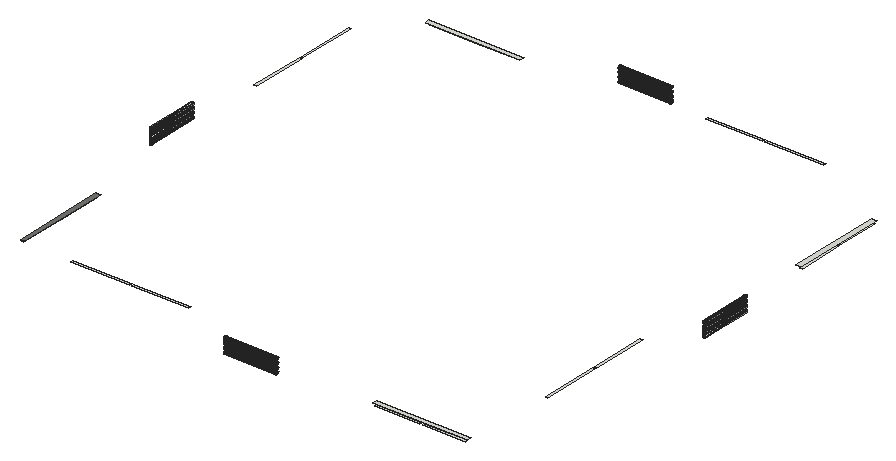
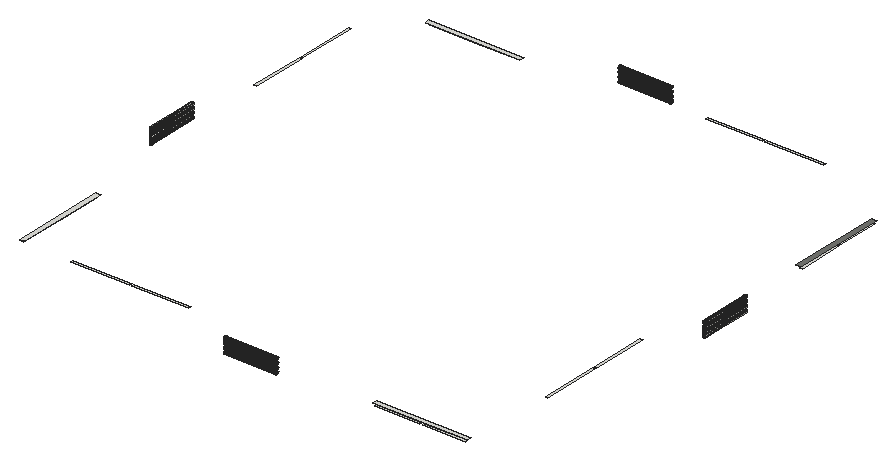
# SketchUp Ruby script. Lengths in inches.
U = 1.inch
M = Sketchup.active_model
def pt(a) = Geom::Point3d.new(a.map { |v| v * U })
def face(e, loops, mat)
  f = e.add_face(loops[0].map { |a| pt(a) })
  loops[1..].each { |l| e.add_face(l.map { |a| pt(a) }).erase! }
  f.material = f.back_material = mat if mat
  f
end
# faces: each face lists its corners as indices into pts; further lists are holes
def faces(e, pts, list, mat = nil) = list.each { |f| face(e, (f[0].is_a?(Array) ? f : [f]).map { |l| l.map { |i| pts[i] } }, mat) }
# xy, xz, yz: faces in a plane at the given z, y or x. An outline is a flat list of corners, or four numbers for a rectangle; further outlines are holes
def ring(l) = l.size == 4 ? [[l[0], l[1]], [l[2], l[1]], [l[2], l[3]], [l[0], l[3]]] : l.each_slice(2).to_a
def flat(e, list, mat, &to3) = list.each { |f| face(e, (f[0].is_a?(Array) ? f : [f]).map { |l| ring(l).map { |u, v| to3.(u, v) } }, mat) }
def xy(e, z, list, mat = nil) = flat(e, list, mat) { |x, y| [x, y, z] }
def xz(e, y, list, mat = nil) = flat(e, list, mat) { |x, z| [x, y, z] }
def yz(e, x, list, mat = nil) = flat(e, list, mat) { |y, z| [x, y, z] }
def lines(e, pts, list) = list.each { |a, b| e.add_line(pt(pts[a]), pt(pts[b])) }
# prism: a flat outline (further loops are holes) pulled along v
def prism(e, loops, v, mat = nil)
  f = face(e, loops, mat); d = Geom::Vector3d.new(v.map { |x| x * U })
  f.pushpull(f.normal.samedirection?(d) ? d.length : -d.length)
end
def box(e, o, s, mat = nil) = prism(e, [[o, [o[0] + s[0], o[1], o[2]], [o[0] + s[0], o[1] + s[1], o[2]], [o[0], o[1] + s[1], o[2]]]], [0, 0, s[2]], mat)
def at(x, y, z, deg = 0) = Geom::Transformation.translation(pt([x, y, z])) * Geom::Transformation.rotation(ORIGIN, Z_AXIS, deg.degrees)
def axes(o, x, y, z) = Geom::Transformation.new([*x, 0, *y, 0, *z, 0, *pt(o).to_a, 1])
def part(name) = M.definitions.add(name)
# library, detail: a bought-in or finely detailed component or shape, given as its bounding box
def library(name, o, s) = part(name).tap { |d| box(d.entities, o, s) }
def detail(e, o, s) = box(e.add_group.entities, o, s)
def put(e, d, t, mat = nil) = e.add_instance(d, t).tap { |i| i.material = mat if mat }
def group(e, t, mat = nil) = e.add_group.tap { |g| g.transformation = t; g.material = mat if mat }.entities
root = M.entities
M.materials.add("[Metal Seamed]").color = [118, 119, 115]
xy(root,1367.61,[[1161.2,84.8125,1285.04,90.8125],[1291.04,84.8125,1408.89,90.8125],[120,175.92,126,293.77],[120,299.77,126,423.61],[1494,1126.01,1500,1249.86],
  [1494,1255.86,1500,1373.7],[211.11,1458.8125,328.96,1464.8125],[334.96,1458.8125,458.8,1464.8125]])
xy(root,1373.61,[[1155.2,84.8125,1414.89,96.8125],[1488,1120.01,1500,1379.7],[205.11,1452.8125,464.8,1464.8125]])
xy(root,1373.61,[[120,169.92,132,429.61]],"[Metal Seamed]")
xy(root,1416.625,[[312.65,102.8125,473.9375,108.8125],[479.9375,102.8125,635.22,108.8125],[1476,277.47,1482,438.75],[1476,444.75,1482,600.03],[138,949.59,144,1104.875],
  [138,1110.875,144,1272.16],[984.78,1440.8125,1140.0625,1446.8125],[1146.0625,1440.8125,1307.35,1446.8125]])
p = [[922.01,48.34,1377.02],[922.01,47.38,1377.14],[778.64,47.38,1377.14],[778.64,48.34,1377.02],[922.01,49.29,1377.14],[778.64,49.29,1377.14],
  [83.53,662.8,1377.02],[82.57,662.8,1377.14],[82.57,806.17,1377.14],[83.53,806.17,1377.02],[84.48,662.8,1377.14],[84.48,806.17,1377.14],
  [1535.52,886.83,1377.14],[1536.47,886.83,1377.02],[1536.47,743.45,1377.02],[1535.52,743.45,1377.14],[1537.43,886.83,1377.14],[1537.43,743.45,1377.14],
  [697.99,1500.33,1377.14],[697.99,1501.28,1377.02],[841.36,1501.28,1377.02],[841.36,1500.33,1377.14],[697.99,1502.24,1377.14],[841.36,1502.24,1377.14],
  [922.01,46.5,1377.51],[778.64,46.5,1377.51],[922.01,50.18,1377.51],[778.64,50.18,1377.51],[81.68,662.8,1377.51],[81.68,806.17,1377.51],
  [85.37,662.8,1377.51],[85.37,806.17,1377.51],[1534.63,886.83,1377.51],[1534.63,743.45,1377.51],[1538.32,886.83,1377.51],[1538.32,743.45,1377.51],
  [697.99,1499.44,1377.51],[841.36,1499.44,1377.51],[697.99,1503.13,1377.51],[841.36,1503.13,1377.51],[922.01,45.73,1378.1],[778.64,45.73,1378.1],
  [922.01,50.95,1378.1],[778.64,50.95,1378.1],[80.92,662.8,1378.1],[80.92,806.17,1378.1],[86.13,662.8,1378.1],[86.13,806.17,1378.1],
  [1533.87,886.83,1378.1],[1533.87,743.45,1378.1],[1539.08,886.83,1378.1],[1539.08,743.45,1378.1],[697.99,1498.68,1378.1],[841.36,1498.68,1378.1],
  [697.99,1503.89,1378.1],[841.36,1503.89,1378.1],[922.01,45.15,1378.86],[778.64,45.15,1378.86],[922.01,51.53,1378.86],[778.64,51.53,1378.86],
  [80.33,662.8,1378.86],[80.33,806.17,1378.86],[86.72,662.8,1378.86],[86.72,806.17,1378.86],[1533.28,886.83,1378.86],[1533.28,743.45,1378.86],
  [1539.67,886.83,1378.86],[1539.67,743.45,1378.86],[697.99,1498.09,1378.86],[841.36,1498.09,1378.86],[697.99,1504.48,1378.86],[841.36,1504.48,1378.86],
  [922.01,44.78,1379.75],[778.64,44.78,1379.75],[922.01,51.9,1379.75],[778.64,51.9,1379.75],[79.97,662.8,1379.75],[79.97,806.17,1379.75],
  [87.09,662.8,1379.75],[87.09,806.17,1379.75],[1532.91,886.83,1379.75],[1532.91,743.45,1379.75],[1540.03,886.83,1379.75],[1540.03,743.45,1379.75],
  [697.99,1497.72,1379.75],[841.36,1497.72,1379.75],[697.99,1504.85,1379.75],[841.36,1504.85,1379.75],[922.01,44.65,1380.7],[778.64,44.65,1380.7],
  [922.01,52.03,1380.7],[778.64,52.03,1380.7],[79.84,662.8,1380.7],[79.84,806.17,1380.7],[87.21,662.8,1380.7],[87.21,806.17,1380.7],
  [1532.79,886.83,1380.7],[1532.79,743.45,1380.7],[1540.16,886.83,1380.7],[1540.16,743.45,1380.7],[697.99,1497.6,1380.7],[841.36,1497.6,1380.7],
  [697.99,1504.97,1380.7],[841.36,1504.97,1380.7],[922.01,44.78,1381.66],[778.64,44.78,1381.66],[922.01,51.9,1381.66],[778.64,51.9,1381.66],
  [79.97,662.8,1381.66],[79.97,806.17,1381.66],[87.09,662.8,1381.66],[87.09,806.17,1381.66],[1532.91,886.83,1381.66],[1532.91,743.45,1381.66],
  [1540.03,886.83,1381.66],[1540.03,743.45,1381.66],[697.99,1497.72,1381.66],[841.36,1497.72,1381.66],[697.99,1504.85,1381.66],[841.36,1504.85,1381.66],
  [922.01,45.15,1382.55],[778.64,45.15,1382.55],[922.01,51.53,1382.55],[778.64,51.53,1382.55],[80.33,662.8,1382.55],[80.33,806.17,1382.55],
  [86.72,662.8,1382.55],[86.72,806.17,1382.55],[1533.28,886.83,1382.55],[1533.28,743.45,1382.55],[1539.67,886.83,1382.55],[1539.67,743.45,1382.55],
  [697.99,1498.09,1382.55],[841.36,1498.09,1382.55],[697.99,1504.48,1382.55],[841.36,1504.48,1382.55],[922.01,45.73,1383.3125],[778.64,45.73,1383.3125],
  [922.01,50.95,1383.3125],[778.64,50.95,1383.3125],[80.92,662.8,1383.3125],[80.92,806.17,1383.3125],[86.13,662.8,1383.3125],[86.13,806.17,1383.3125],
  [1533.87,886.83,1383.3125],[1533.87,743.45,1383.3125],[1539.08,886.83,1383.3125],[1539.08,743.45,1383.3125],[697.99,1498.68,1383.3125],[841.36,1498.68,1383.3125],
  [697.99,1503.89,1383.3125],[841.36,1503.89,1383.3125],[922.01,46.5,1383.9],[778.64,46.5,1383.9],[922.01,50.18,1383.9],[778.64,50.18,1383.9],
  [81.68,662.8,1383.9],[81.68,806.17,1383.9],[85.37,662.8,1383.9],[85.37,806.17,1383.9],[1534.63,886.83,1383.9],[1534.63,743.45,1383.9],
  [1538.32,886.83,1383.9],[1538.32,743.45,1383.9],[697.99,1499.44,1383.9],[841.36,1499.44,1383.9],[697.99,1503.13,1383.9],[841.36,1503.13,1383.9],
  [922.01,47.38,1384.27],[778.64,47.38,1384.27],[922.01,49.29,1384.27],[778.64,49.29,1384.27],[82.57,662.8,1384.27],[82.57,806.17,1384.27],
  [84.48,662.8,1384.27],[84.48,806.17,1384.27],[1535.52,886.83,1384.27],[1535.52,743.45,1384.27],[1537.43,886.83,1384.27],[1537.43,743.45,1384.27],
  [697.99,1500.33,1384.27],[841.36,1500.33,1384.27],[697.99,1502.24,1384.27],[841.36,1502.24,1384.27],[922.01,48.34,1384.39],[778.64,48.34,1384.39],
  [83.53,662.8,1384.39],[83.53,806.17,1384.39],[1536.47,886.83,1384.39],[1536.47,743.45,1384.39],[697.99,1501.28,1384.39],[841.36,1501.28,1384.39],
  [922.01,48.34,1389.02],[922.01,47.38,1389.14],[778.64,47.38,1389.14],[778.64,48.34,1389.02],[922.01,49.29,1389.14],[778.64,49.29,1389.14],
  [83.53,662.8,1389.02],[82.57,662.8,1389.14],[82.57,806.17,1389.14],[83.53,806.17,1389.02],[84.48,662.8,1389.14],[84.48,806.17,1389.14],
  [1535.52,886.83,1389.14],[1536.47,886.83,1389.02],[1536.47,743.45,1389.02],[1535.52,743.45,1389.14],[1537.43,886.83,1389.14],[1537.43,743.45,1389.14],
  [697.99,1500.33,1389.14],[697.99,1501.28,1389.02],[841.36,1501.28,1389.02],[841.36,1500.33,1389.14],[697.99,1502.24,1389.14],[841.36,1502.24,1389.14],
  [922.01,46.5,1389.51],[778.64,46.5,1389.51],[922.01,50.18,1389.51],[778.64,50.18,1389.51],[81.68,662.8,1389.51],[81.68,806.17,1389.51],
  [85.37,662.8,1389.51],[85.37,806.17,1389.51],[1534.63,886.83,1389.51],[1534.63,743.45,1389.51],[1538.32,886.83,1389.51],[1538.32,743.45,1389.51],
  [697.99,1499.44,1389.51],[841.36,1499.44,1389.51],[697.99,1503.13,1389.51],[841.36,1503.13,1389.51],[922.01,45.73,1390.1],[778.64,45.73,1390.1],
  [922.01,50.95,1390.1],[778.64,50.95,1390.1],[80.92,662.8,1390.1],[80.92,806.17,1390.1],[86.13,662.8,1390.1],[86.13,806.17,1390.1],
  [1533.87,886.83,1390.1],[1533.87,743.45,1390.1],[1539.08,886.83,1390.1],[1539.08,743.45,1390.1],[697.99,1498.68,1390.1],[841.36,1498.68,1390.1],
  [697.99,1503.89,1390.1],[841.36,1503.89,1390.1],[922.01,45.15,1390.86],[778.64,45.15,1390.86],[922.01,51.53,1390.86],[778.64,51.53,1390.86],
  [80.33,662.8,1390.86],[80.33,806.17,1390.86],[86.72,662.8,1390.86],[86.72,806.17,1390.86],[1533.28,886.83,1390.86],[1533.28,743.45,1390.86],
  [1539.67,886.83,1390.86],[1539.67,743.45,1390.86],[697.99,1498.09,1390.86],[841.36,1498.09,1390.86],[697.99,1504.48,1390.86],[841.36,1504.48,1390.86],
  [922.01,44.78,1391.75],[778.64,44.78,1391.75],[922.01,51.9,1391.75],[778.64,51.9,1391.75],[79.97,662.8,1391.75],[79.97,806.17,1391.75],
  [87.09,662.8,1391.75],[87.09,806.17,1391.75],[1532.91,886.83,1391.75],[1532.91,743.45,1391.75],[1540.03,886.83,1391.75],[1540.03,743.45,1391.75],
  [697.99,1497.72,1391.75],[841.36,1497.72,1391.75],[697.99,1504.85,1391.75],[841.36,1504.85,1391.75],[922.01,44.65,1392.7],[778.64,44.65,1392.7],
  [922.01,52.03,1392.7],[778.64,52.03,1392.7],[79.84,662.8,1392.7],[79.84,806.17,1392.7],[87.21,662.8,1392.7],[87.21,806.17,1392.7],
  [1532.79,886.83,1392.7],[1532.79,743.45,1392.7],[1540.16,886.83,1392.7],[1540.16,743.45,1392.7],[697.99,1497.6,1392.7],[841.36,1497.6,1392.7],
  [697.99,1504.97,1392.7],[841.36,1504.97,1392.7],[922.01,44.78,1393.66],[778.64,44.78,1393.66],[922.01,51.9,1393.66],[778.64,51.9,1393.66],
  [79.97,662.8,1393.66],[79.97,806.17,1393.66],[87.09,662.8,1393.66],[87.09,806.17,1393.66],[1532.91,886.83,1393.66],[1532.91,743.45,1393.66],
  [1540.03,886.83,1393.66],[1540.03,743.45,1393.66],[697.99,1497.72,1393.66],[841.36,1497.72,1393.66],[697.99,1504.85,1393.66],[841.36,1504.85,1393.66],
  [922.01,45.15,1394.55],[778.64,45.15,1394.55],[922.01,51.53,1394.55],[778.64,51.53,1394.55],[80.33,662.8,1394.55],[80.33,806.17,1394.55],
  [86.72,662.8,1394.55],[86.72,806.17,1394.55],[1533.28,886.83,1394.55],[1533.28,743.45,1394.55],[1539.67,886.83,1394.55],[1539.67,743.45,1394.55],
  [697.99,1498.09,1394.55],[841.36,1498.09,1394.55],[697.99,1504.48,1394.55],[841.36,1504.48,1394.55],[922.01,45.73,1395.3125],[778.64,45.73,1395.3125],
  [922.01,50.95,1395.3125],[778.64,50.95,1395.3125],[80.92,662.8,1395.3125],[80.92,806.17,1395.3125],[86.13,662.8,1395.3125],[86.13,806.17,1395.3125],
  [1533.87,886.83,1395.3125],[1533.87,743.45,1395.3125],[1539.08,886.83,1395.3125],[1539.08,743.45,1395.3125],[697.99,1498.68,1395.3125],[841.36,1498.68,1395.3125],
  [697.99,1503.89,1395.3125],[841.36,1503.89,1395.3125],[922.01,46.5,1395.9],[778.64,46.5,1395.9],[922.01,50.18,1395.9],[778.64,50.18,1395.9],
  [81.68,662.8,1395.9],[81.68,806.17,1395.9],[85.37,662.8,1395.9],[85.37,806.17,1395.9],[1534.63,886.83,1395.9],[1534.63,743.45,1395.9],
  [1538.32,886.83,1395.9],[1538.32,743.45,1395.9],[697.99,1499.44,1395.9],[841.36,1499.44,1395.9],[697.99,1503.13,1395.9],[841.36,1503.13,1395.9],
  [922.01,47.38,1396.27],[778.64,47.38,1396.27],[922.01,49.29,1396.27],[778.64,49.29,1396.27],[82.57,662.8,1396.27],[82.57,806.17,1396.27],
  [84.48,662.8,1396.27],[84.48,806.17,1396.27],[1535.52,886.83,1396.27],[1535.52,743.45,1396.27],[1537.43,886.83,1396.27],[1537.43,743.45,1396.27],
  [697.99,1500.33,1396.27],[841.36,1500.33,1396.27],[697.99,1502.24,1396.27],[841.36,1502.24,1396.27],[922.01,48.34,1396.39],[778.64,48.34,1396.39],
  [83.53,662.8,1396.39],[83.53,806.17,1396.39],[1536.47,886.83,1396.39],[1536.47,743.45,1396.39],[697.99,1501.28,1396.39],[841.36,1501.28,1396.39],
  [922.01,48.34,1401.02],[922.01,47.38,1401.14],[778.64,47.38,1401.14],[778.64,48.34,1401.02],[922.01,49.29,1401.14],[778.64,49.29,1401.14],
  [83.53,662.8,1401.02],[82.57,662.8,1401.14],[82.57,806.17,1401.14],[83.53,806.17,1401.02],[84.48,662.8,1401.14],[84.48,806.17,1401.14],
  [1535.52,886.83,1401.14],[1536.47,886.83,1401.02],[1536.47,743.45,1401.02],[1535.52,743.45,1401.14],[1537.43,886.83,1401.14],[1537.43,743.45,1401.14],
  [697.99,1500.33,1401.14],[697.99,1501.28,1401.02],[841.36,1501.28,1401.02],[841.36,1500.33,1401.14],[697.99,1502.24,1401.14],[841.36,1502.24,1401.14],
  [922.01,46.5,1401.51],[778.64,46.5,1401.51],[922.01,50.18,1401.51],[778.64,50.18,1401.51],[81.68,662.8,1401.51],[81.68,806.17,1401.51],
  [85.37,662.8,1401.51],[85.37,806.17,1401.51],[1534.63,886.83,1401.51],[1534.63,743.45,1401.51],[1538.32,886.83,1401.51],[1538.32,743.45,1401.51],
  [697.99,1499.44,1401.51],[841.36,1499.44,1401.51],[697.99,1503.13,1401.51],[841.36,1503.13,1401.51],[922.01,45.73,1402.1],[778.64,45.73,1402.1],
  [922.01,50.95,1402.1],[778.64,50.95,1402.1],[80.92,662.8,1402.1],[80.92,806.17,1402.1],[86.13,662.8,1402.1],[86.13,806.17,1402.1],
  [1533.87,886.83,1402.1],[1533.87,743.45,1402.1],[1539.08,886.83,1402.1],[1539.08,743.45,1402.1],[697.99,1498.68,1402.1],[841.36,1498.68,1402.1],
  [697.99,1503.89,1402.1],[841.36,1503.89,1402.1],[922.01,45.15,1402.86],[778.64,45.15,1402.86],[922.01,51.53,1402.86],[778.64,51.53,1402.86],
  [80.33,662.8,1402.86],[80.33,806.17,1402.86],[86.72,662.8,1402.86],[86.72,806.17,1402.86],[1533.28,886.83,1402.86],[1533.28,743.45,1402.86],
  [1539.67,886.83,1402.86],[1539.67,743.45,1402.86],[697.99,1498.09,1402.86],[841.36,1498.09,1402.86],[697.99,1504.48,1402.86],[841.36,1504.48,1402.86],
  [922.01,44.78,1403.75],[778.64,44.78,1403.75],[922.01,51.9,1403.75],[778.64,51.9,1403.75],[79.97,662.8,1403.75],[79.97,806.17,1403.75],
  [87.09,662.8,1403.75],[87.09,806.17,1403.75],[1532.91,886.83,1403.75],[1532.91,743.45,1403.75],[1540.03,886.83,1403.75],[1540.03,743.45,1403.75],
  [697.99,1497.72,1403.75],[841.36,1497.72,1403.75],[697.99,1504.85,1403.75],[841.36,1504.85,1403.75],[922.01,44.65,1404.7],[778.64,44.65,1404.7],
  [922.01,52.03,1404.7],[778.64,52.03,1404.7],[79.84,662.8,1404.7],[79.84,806.17,1404.7],[87.21,662.8,1404.7],[87.21,806.17,1404.7],
  [1532.79,886.83,1404.7],[1532.79,743.45,1404.7],[1540.16,886.83,1404.7],[1540.16,743.45,1404.7],[697.99,1497.6,1404.7],[841.36,1497.6,1404.7],
  [697.99,1504.97,1404.7],[841.36,1504.97,1404.7],[922.01,44.78,1405.66],[778.64,44.78,1405.66],[922.01,51.9,1405.66],[778.64,51.9,1405.66],
  [79.97,662.8,1405.66],[79.97,806.17,1405.66],[87.09,662.8,1405.66],[87.09,806.17,1405.66],[1532.91,886.83,1405.66],[1532.91,743.45,1405.66],
  [1540.03,886.83,1405.66],[1540.03,743.45,1405.66],[697.99,1497.72,1405.66],[841.36,1497.72,1405.66],[697.99,1504.85,1405.66],[841.36,1504.85,1405.66],
  [922.01,45.15,1406.55],[778.64,45.15,1406.55],[922.01,51.53,1406.55],[778.64,51.53,1406.55],[80.33,662.8,1406.55],[80.33,806.17,1406.55],
  [86.72,662.8,1406.55],[86.72,806.17,1406.55],[1533.28,886.83,1406.55],[1533.28,743.45,1406.55],[1539.67,886.83,1406.55],[1539.67,743.45,1406.55],
  [697.99,1498.09,1406.55],[841.36,1498.09,1406.55],[697.99,1504.48,1406.55],[841.36,1504.48,1406.55],[922.01,45.73,1407.3125],[778.64,45.73,1407.3125],
  [922.01,50.95,1407.3125],[778.64,50.95,1407.3125],[80.92,662.8,1407.3125],[80.92,806.17,1407.3125],[86.13,662.8,1407.3125],[86.13,806.17,1407.3125],
  [1533.87,886.83,1407.3125],[1533.87,743.45,1407.3125],[1539.08,886.83,1407.3125],[1539.08,743.45,1407.3125],[697.99,1498.68,1407.3125],[841.36,1498.68,1407.3125],
  [697.99,1503.89,1407.3125],[841.36,1503.89,1407.3125],[922.01,46.5,1407.9],[778.64,46.5,1407.9],[922.01,50.18,1407.9],[778.64,50.18,1407.9],
  [81.68,662.8,1407.9],[81.68,806.17,1407.9],[85.37,662.8,1407.9],[85.37,806.17,1407.9],[1534.63,886.83,1407.9],[1534.63,743.45,1407.9],
  [1538.32,886.83,1407.9],[1538.32,743.45,1407.9],[697.99,1499.44,1407.9],[841.36,1499.44,1407.9],[697.99,1503.13,1407.9],[841.36,1503.13,1407.9],
  [922.01,47.38,1408.27],[778.64,47.38,1408.27],[922.01,49.29,1408.27],[778.64,49.29,1408.27],[82.57,662.8,1408.27],[82.57,806.17,1408.27],
  [84.48,662.8,1408.27],[84.48,806.17,1408.27],[1535.52,886.83,1408.27],[1535.52,743.45,1408.27],[1537.43,886.83,1408.27],[1537.43,743.45,1408.27],
  [697.99,1500.33,1408.27],[841.36,1500.33,1408.27],[697.99,1502.24,1408.27],[841.36,1502.24,1408.27],[922.01,48.34,1408.39],[778.64,48.34,1408.39],
  [83.53,662.8,1408.39],[83.53,806.17,1408.39],[1536.47,886.83,1408.39],[1536.47,743.45,1408.39],[697.99,1501.28,1408.39],[841.36,1501.28,1408.39],
  [922.01,48.34,1413.02],[922.01,47.38,1413.14],[778.64,47.38,1413.14],[778.64,48.34,1413.02],[922.01,49.29,1413.14],[778.64,49.29,1413.14],
  [83.53,662.8,1413.02],[82.57,662.8,1413.14],[82.57,806.17,1413.14],[83.53,806.17,1413.02],[84.48,662.8,1413.14],[84.48,806.17,1413.14],
  [1535.52,886.83,1413.14],[1536.47,886.83,1413.02],[1536.47,743.45,1413.02],[1535.52,743.45,1413.14],[1537.43,886.83,1413.14],[1537.43,743.45,1413.14],
  [697.99,1500.33,1413.14],[697.99,1501.28,1413.02],[841.36,1501.28,1413.02],[841.36,1500.33,1413.14],[697.99,1502.24,1413.14],[841.36,1502.24,1413.14],
  [922.01,46.5,1413.51],[778.64,46.5,1413.51],[922.01,50.18,1413.51],[778.64,50.18,1413.51],[81.68,662.8,1413.51],[81.68,806.17,1413.51],
  [85.37,662.8,1413.51],[85.37,806.17,1413.51],[1534.63,886.83,1413.51],[1534.63,743.45,1413.51],[1538.32,886.83,1413.51],[1538.32,743.45,1413.51],
  [697.99,1499.44,1413.51],[841.36,1499.44,1413.51],[697.99,1503.13,1413.51],[841.36,1503.13,1413.51],[922.01,45.73,1414.1],[778.64,45.73,1414.1],
  [922.01,50.95,1414.1],[778.64,50.95,1414.1],[80.92,662.8,1414.1],[80.92,806.17,1414.1],[86.13,662.8,1414.1],[86.13,806.17,1414.1],
  [1533.87,886.83,1414.1],[1533.87,743.45,1414.1],[1539.08,886.83,1414.1],[1539.08,743.45,1414.1],[697.99,1498.68,1414.1],[841.36,1498.68,1414.1],
  [697.99,1503.89,1414.1],[841.36,1503.89,1414.1],[922.01,45.15,1414.86],[778.64,45.15,1414.86],[922.01,51.53,1414.86],[778.64,51.53,1414.86],
  [80.33,662.8,1414.86],[80.33,806.17,1414.86],[86.72,662.8,1414.86],[86.72,806.17,1414.86],[1533.28,886.83,1414.86],[1533.28,743.45,1414.86],
  [1539.67,886.83,1414.86],[1539.67,743.45,1414.86],[697.99,1498.09,1414.86],[841.36,1498.09,1414.86],[697.99,1504.48,1414.86],[841.36,1504.48,1414.86],
  [922.01,44.78,1415.75],[778.64,44.78,1415.75],[922.01,51.9,1415.75],[778.64,51.9,1415.75],[79.97,662.8,1415.75],[79.97,806.17,1415.75],
  [87.09,662.8,1415.75],[87.09,806.17,1415.75],[1532.91,886.83,1415.75],[1532.91,743.45,1415.75],[1540.03,886.83,1415.75],[1540.03,743.45,1415.75],
  [697.99,1497.72,1415.75],[841.36,1497.72,1415.75],[697.99,1504.85,1415.75],[841.36,1504.85,1415.75],[922.01,44.65,1416.7],[778.64,44.65,1416.7],
  [922.01,52.03,1416.7],[778.64,52.03,1416.7],[79.84,662.8,1416.7],[79.84,806.17,1416.7],[87.21,662.8,1416.7],[87.21,806.17,1416.7],
  [1532.79,886.83,1416.7],[1532.79,743.45,1416.7],[1540.16,886.83,1416.7],[1540.16,743.45,1416.7],[697.99,1497.6,1416.7],[841.36,1497.6,1416.7],
  [697.99,1504.97,1416.7],[841.36,1504.97,1416.7],[922.01,44.78,1417.66],[778.64,44.78,1417.66],[922.01,51.9,1417.66],[778.64,51.9,1417.66],
  [79.97,662.8,1417.66],[79.97,806.17,1417.66],[87.09,662.8,1417.66],[87.09,806.17,1417.66],[1532.91,886.83,1417.66],[1532.91,743.45,1417.66],
  [1540.03,886.83,1417.66],[1540.03,743.45,1417.66],[697.99,1497.72,1417.66],[841.36,1497.72,1417.66],[697.99,1504.85,1417.66],[841.36,1504.85,1417.66],
  [922.01,45.15,1418.55],[778.64,45.15,1418.55],[922.01,51.53,1418.55],[778.64,51.53,1418.55],[80.33,662.8,1418.55],[80.33,806.17,1418.55],
  [86.72,662.8,1418.55],[86.72,806.17,1418.55],[1533.28,886.83,1418.55],[1533.28,743.45,1418.55],[1539.67,886.83,1418.55],[1539.67,743.45,1418.55],
  [697.99,1498.09,1418.55],[841.36,1498.09,1418.55],[697.99,1504.48,1418.55],[841.36,1504.48,1418.55],[922.01,45.73,1419.3125],[778.64,45.73,1419.3125],
  [922.01,50.95,1419.3125],[778.64,50.95,1419.3125],[80.92,662.8,1419.3125],[80.92,806.17,1419.3125],[86.13,662.8,1419.3125],[86.13,806.17,1419.3125],
  [1533.87,886.83,1419.3125],[1533.87,743.45,1419.3125],[1539.08,886.83,1419.3125],[1539.08,743.45,1419.3125],[697.99,1498.68,1419.3125],[841.36,1498.68,1419.3125],
  [697.99,1503.89,1419.3125],[841.36,1503.89,1419.3125],[922.01,46.5,1419.9],[778.64,46.5,1419.9],[922.01,50.18,1419.9],[778.64,50.18,1419.9],
  [81.68,662.8,1419.9],[81.68,806.17,1419.9],[85.37,662.8,1419.9],[85.37,806.17,1419.9],[1534.63,886.83,1419.9],[1534.63,743.45,1419.9],
  [1538.32,886.83,1419.9],[1538.32,743.45,1419.9],[697.99,1499.44,1419.9],[841.36,1499.44,1419.9],[697.99,1503.13,1419.9],[841.36,1503.13,1419.9],
  [922.01,47.38,1420.27],[778.64,47.38,1420.27],[922.01,49.29,1420.27],[778.64,49.29,1420.27],[82.57,662.8,1420.27],[82.57,806.17,1420.27],
  [84.48,662.8,1420.27],[84.48,806.17,1420.27],[1535.52,886.83,1420.27],[1535.52,743.45,1420.27],[1537.43,886.83,1420.27],[1537.43,743.45,1420.27],
  [697.99,1500.33,1420.27],[841.36,1500.33,1420.27],[697.99,1502.24,1420.27],[841.36,1502.24,1420.27],[922.01,48.34,1420.39],[778.64,48.34,1420.39],
  [83.53,662.8,1420.39],[83.53,806.17,1420.39],[1536.47,886.83,1420.39],[1536.47,743.45,1420.39],[697.99,1501.28,1420.39],[841.36,1501.28,1420.39]]
faces(root,p,[[0,1,2,3],[4,0,3,5],[6,7,8,9],[10,6,9,11],[12,13,14,15],[13,16,17,14],[18,19,20,21],[19,22,23,20],
  [1,24,25,2],[26,4,5,27],[7,28,29,8],[30,10,11,31],[32,12,15,33],[16,34,35,17],[36,18,21,37],[22,38,39,23],
  [24,40,41,25],[42,26,27,43],[28,44,45,29],[46,30,31,47],[48,32,33,49],[34,50,51,35],[52,36,37,53],[38,54,55,39],
  [40,56,57,41],[58,42,43,59],[44,60,61,45],[62,46,47,63],[64,48,49,65],[50,66,67,51],[68,52,53,69],[54,70,71,55],
  [56,72,73,57],[74,58,59,75],[60,76,77,61],[78,62,63,79],[80,64,65,81],[66,82,83,67],[84,68,69,85],[70,86,87,71],
  [72,88,89,73],[90,74,75,91],[76,92,93,77],[94,78,79,95],[96,80,81,97],[82,98,99,83],[100,84,85,101],[86,102,103,87],
  [88,104,105,89],[106,90,91,107],[92,108,109,93],[110,94,95,111],[112,96,97,113],[98,114,115,99],[116,100,101,117],[102,118,119,103],
  [104,120,121,105],[122,106,107,123],[108,124,125,109],[126,110,111,127],[128,112,113,129],[114,130,131,115],[132,116,117,133],[118,134,135,119],
  [120,136,137,121],[138,122,123,139],[124,140,141,125],[142,126,127,143],[144,128,129,145],[130,146,147,131],[148,132,133,149],[134,150,151,135],
  [136,152,153,137],[154,138,139,155],[140,156,157,141],[158,142,143,159],[160,144,145,161],[146,162,163,147],[164,148,149,165],[150,166,167,151],
  [152,168,169,153],[170,154,155,171],[156,172,173,157],[174,158,159,175],[176,160,161,177],[162,178,179,163],[180,164,165,181],[166,182,183,167],
  [168,184,185,169],[184,170,171,185],[172,186,187,173],[186,174,175,187],[188,176,177,189],[178,188,189,179],[190,180,181,191],[182,190,191,183],
  [192,193,194,195],[196,192,195,197],[198,199,200,201],[202,198,201,203],[204,205,206,207],[205,208,209,206],[210,211,212,213],[211,214,215,212],
  [193,216,217,194],[218,196,197,219],[199,220,221,200],[222,202,203,223],[224,204,207,225],[208,226,227,209],[228,210,213,229],[214,230,231,215],
  [216,232,233,217],[234,218,219,235],[220,236,237,221],[238,222,223,239],[240,224,225,241],[226,242,243,227],[244,228,229,245],[230,246,247,231],
  [232,248,249,233],[250,234,235,251],[236,252,253,237],[254,238,239,255],[256,240,241,257],[242,258,259,243],[260,244,245,261],[246,262,263,247],
  [248,264,265,249],[266,250,251,267],[252,268,269,253],[270,254,255,271],[272,256,257,273],[258,274,275,259],[276,260,261,277],[262,278,279,263],
  [264,280,281,265],[282,266,267,283],[268,284,285,269],[286,270,271,287],[288,272,273,289],[274,290,291,275],[292,276,277,293],[278,294,295,279],
  [280,296,297,281],[298,282,283,299],[284,300,301,285],[302,286,287,303],[304,288,289,305],[290,306,307,291],[308,292,293,309],[294,310,311,295],
  [296,312,313,297],[314,298,299,315],[300,316,317,301],[318,302,303,319],[320,304,305,321],[306,322,323,307],[324,308,309,325],[310,326,327,311],
  [312,328,329,313],[330,314,315,331],[316,332,333,317],[334,318,319,335],[336,320,321,337],[322,338,339,323],[340,324,325,341],[326,342,343,327],
  [328,344,345,329],[346,330,331,347],[332,348,349,333],[350,334,335,351],[352,336,337,353],[338,354,355,339],[356,340,341,357],[342,358,359,343],
  [344,360,361,345],[362,346,347,363],[348,364,365,349],[366,350,351,367],[368,352,353,369],[354,370,371,355],[372,356,357,373],[358,374,375,359],
  [360,376,377,361],[376,362,363,377],[364,378,379,365],[378,366,367,379],[380,368,369,381],[370,380,381,371],[382,372,373,383],[374,382,383,375],
  [384,385,386,387],[388,384,387,389],[390,391,392,393],[394,390,393,395],[396,397,398,399],[397,400,401,398],[402,403,404,405],[403,406,407,404],
  [385,408,409,386],[410,388,389,411],[391,412,413,392],[414,394,395,415],[416,396,399,417],[400,418,419,401],[420,402,405,421],[406,422,423,407],
  [408,424,425,409],[426,410,411,427],[412,428,429,413],[430,414,415,431],[432,416,417,433],[418,434,435,419],[436,420,421,437],[422,438,439,423],
  [424,440,441,425],[442,426,427,443],[428,444,445,429],[446,430,431,447],[448,432,433,449],[434,450,451,435],[452,436,437,453],[438,454,455,439],
  [440,456,457,441],[458,442,443,459],[444,460,461,445],[462,446,447,463],[464,448,449,465],[450,466,467,451],[468,452,453,469],[454,470,471,455],
  [456,472,473,457],[474,458,459,475],[460,476,477,461],[478,462,463,479],[480,464,465,481],[466,482,483,467],[484,468,469,485],[470,486,487,471],
  [472,488,489,473],[490,474,475,491],[476,492,493,477],[494,478,479,495],[496,480,481,497],[482,498,499,483],[500,484,485,501],[486,502,503,487],
  [488,504,505,489],[506,490,491,507],[492,508,509,493],[510,494,495,511],[512,496,497,513],[498,514,515,499],[516,500,501,517],[502,518,519,503],
  [504,520,521,505],[522,506,507,523],[508,524,525,509],[526,510,511,527],[528,512,513,529],[514,530,531,515],[532,516,517,533],[518,534,535,519],
  [520,536,537,521],[538,522,523,539],[524,540,541,525],[542,526,527,543],[544,528,529,545],[530,546,547,531],[548,532,533,549],[534,550,551,535],
  [536,552,553,537],[554,538,539,555],[540,556,557,541],[558,542,543,559],[560,544,545,561],[546,562,563,547],[564,548,549,565],[550,566,567,551],
  [552,568,569,553],[568,554,555,569],[556,570,571,557],[570,558,559,571],[572,560,561,573],[562,572,573,563],[574,564,565,575],[566,574,575,567],
  [576,577,578,579],[580,576,579,581],[582,583,584,585],[586,582,585,587],[588,589,590,591],[589,592,593,590],[594,595,596,597],[595,598,599,596],
  [577,600,601,578],[602,580,581,603],[583,604,605,584],[606,586,587,607],[608,588,591,609],[592,610,611,593],[612,594,597,613],[598,614,615,599],
  [600,616,617,601],[618,602,603,619],[604,620,621,605],[622,606,607,623],[624,608,609,625],[610,626,627,611],[628,612,613,629],[614,630,631,615],
  [616,632,633,617],[634,618,619,635],[620,636,637,621],[638,622,623,639],[640,624,625,641],[626,642,643,627],[644,628,629,645],[630,646,647,631],
  [632,648,649,633],[650,634,635,651],[636,652,653,637],[654,638,639,655],[656,640,641,657],[642,658,659,643],[660,644,645,661],[646,662,663,647],
  [648,664,665,649],[666,650,651,667],[652,668,669,653],[670,654,655,671],[672,656,657,673],[658,674,675,659],[676,660,661,677],[662,678,679,663],
  [664,680,681,665],[682,666,667,683],[668,684,685,669],[686,670,671,687],[688,672,673,689],[674,690,691,675],[692,676,677,693],[678,694,695,679],
  [680,696,697,681],[698,682,683,699],[684,700,701,685],[702,686,687,703],[704,688,689,705],[690,706,707,691],[708,692,693,709],[694,710,711,695],
  [696,712,713,697],[714,698,699,715],[700,716,717,701],[718,702,703,719],[720,704,705,721],[706,722,723,707],[724,708,709,725],[710,726,727,711],
  [712,728,729,713],[730,714,715,731],[716,732,733,717],[734,718,719,735],[736,720,721,737],[722,738,739,723],[740,724,725,741],[726,742,743,727],
  [728,744,745,729],[746,730,731,747],[732,748,749,733],[750,734,735,751],[752,736,737,753],[738,754,755,739],[756,740,741,757],[742,758,759,743],
  [744,760,761,745],[760,746,747,761],[748,762,763,749],[762,750,751,763],[764,752,753,765],[754,764,765,755],[766,756,757,767],[758,766,767,759]])
